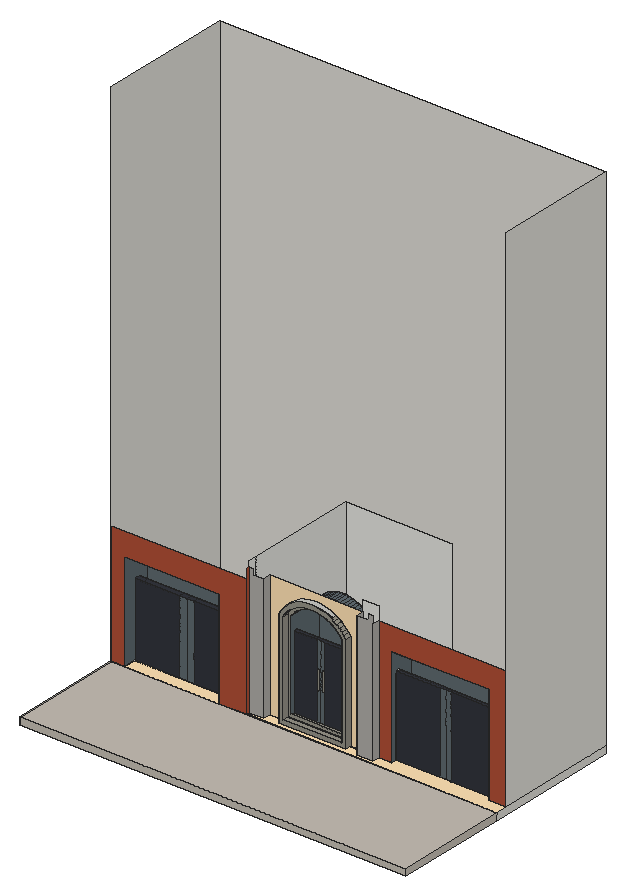
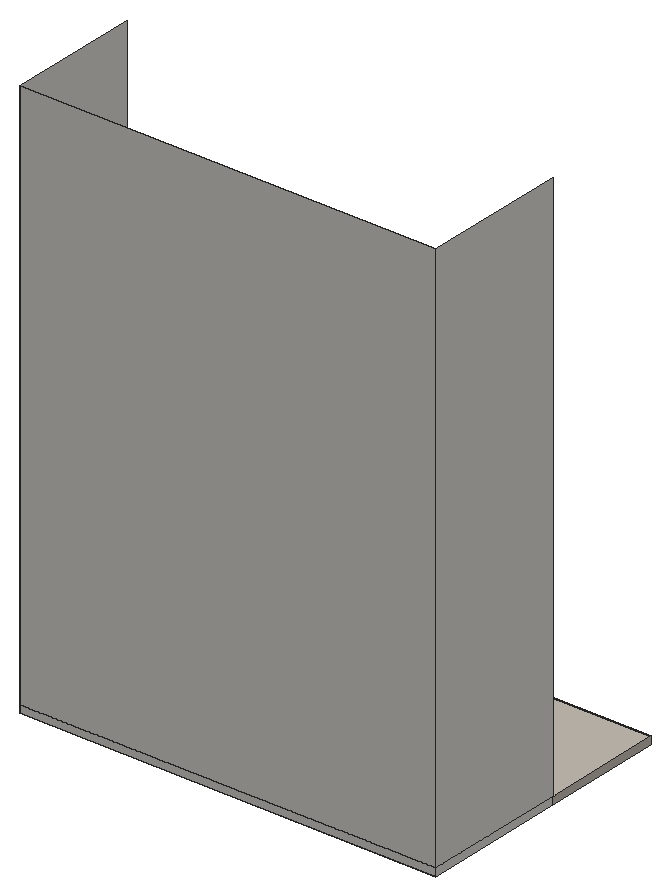
# SketchUp Ruby script. Lengths in inches.
U = 1.inch
M = Sketchup.active_model
def pt(a) = Geom::Point3d.new(a.map { |v| v * U })
def face(e, loops, mat)
  f = e.add_face(loops[0].map { |a| pt(a) })
  loops[1..].each { |l| e.add_face(l.map { |a| pt(a) }).erase! }
  f.material = f.back_material = mat if mat
  f
end
# faces: each face lists its corners as indices into pts; further lists are holes
def faces(e, pts, list, mat = nil) = list.each { |f| face(e, (f[0].is_a?(Array) ? f : [f]).map { |l| l.map { |i| pts[i] } }, mat) }
# xy, xz, yz: faces in a plane at the given z, y or x. An outline is a flat list of corners, or four numbers for a rectangle; further outlines are holes
def ring(l) = l.size == 4 ? [[l[0], l[1]], [l[2], l[1]], [l[2], l[3]], [l[0], l[3]]] : l.each_slice(2).to_a
def flat(e, list, mat, &to3) = list.each { |f| face(e, (f[0].is_a?(Array) ? f : [f]).map { |l| ring(l).map { |u, v| to3.(u, v) } }, mat) }
def xy(e, z, list, mat = nil) = flat(e, list, mat) { |x, y| [x, y, z] }
def xz(e, y, list, mat = nil) = flat(e, list, mat) { |x, z| [x, y, z] }
def yz(e, x, list, mat = nil) = flat(e, list, mat) { |y, z| [x, y, z] }
def lines(e, pts, list) = list.each { |a, b| e.add_line(pt(pts[a]), pt(pts[b])) }
# prism: a flat outline (further loops are holes) pulled along v
def prism(e, loops, v, mat = nil)
  f = face(e, loops, mat); d = Geom::Vector3d.new(v.map { |x| x * U })
  f.pushpull(f.normal.samedirection?(d) ? d.length : -d.length)
end
def box(e, o, s, mat = nil) = prism(e, [[o, [o[0] + s[0], o[1], o[2]], [o[0] + s[0], o[1] + s[1], o[2]], [o[0], o[1] + s[1], o[2]]]], [0, 0, s[2]], mat)
def at(x, y, z, deg = 0) = Geom::Transformation.translation(pt([x, y, z])) * Geom::Transformation.rotation(ORIGIN, Z_AXIS, deg.degrees)
def axes(o, x, y, z) = Geom::Transformation.new([*x, 0, *y, 0, *z, 0, *pt(o).to_a, 1])
def part(name) = M.definitions.add(name)
# library, detail: a bought-in or finely detailed component or shape, given as its bounding box
def library(name, o, s) = part(name).tap { |d| box(d.entities, o, s) }
def detail(e, o, s) = box(e.add_group.entities, o, s)
def put(e, d, t, mat = nil) = e.add_instance(d, t).tap { |i| i.material = mat if mat }
def group(e, t, mat = nil) = e.add_group.tap { |g| g.transformation = t; g.material = mat if mat }.entities
root = M.entities
M.materials.add("[Field Rectangle Tile]").color = [196, 189, 179]
M.materials.add("[Formica Beige]").color = [255, 225, 180]
M.materials.add("[Formica Graystone]").color = [149, 146, 135]
M.materials.add("[Formica Laminate Dark]").color = [50, 53, 60]
M.materials.add("[Formica Speckled Grey]").color = [94, 105, 111]
M.materials.add("[Rough Square Concrete Block]").color = [175, 79, 54]
M.materials.add("[Terrazzo Tile Light]").color = [173, 171, 166]
M.materials.add("[Terrazzo Tile Light]1").color = [219, 217, 210]
xy(root,0,[[10.25,0,499.12,144.04],[10.25,144.04,10.25,315.41,499.12,315.41,499.12,144.04,146.29,144.04,146.29,178.85,26.98,178.85,26.98,167.22,37.92,167.22,37.92,159.93,26.98,159.93,26.98,144.04],[26.98,144.04,146.29,159.93],[37.92,159.93,146.29,167.22],[26.98,167.22,146.29,178.85]])
xy(root,9,[[181.54,148.61,199.67,158.3],[317.75,148.61,338.35,158.3],[217.06,150.74,302.12,158.3],[181.54,158.3,181.54,301.14,315.73,301.14,338.35,158.3],[338.35,158.3,315.73,301.14,449.92,301.14,449.92,187.55,354.68,187.55,354.68,158.3],
  [354.68,164.83,476.62,168.86],[354.68,168.86,476.62,187.55]])
xy(root,9,[[10.25,0,499.12,144.04]],"[Field Rectangle Tile]")
xy(root,9,[[26.98,144.04,146.29,159.93],[181.54,144.04,499.12,144.04,499.12,158.3,476.62,158.3,476.62,164.83,354.68,164.83,354.68,158.3,338.35,158.3,338.35,148.61,317.75,148.61,317.75,158.3,302.12,158.3,302.12,150.74,217.06,150.74,217.06,158.3,199.67,158.3,199.67,148.61,181.54,148.61]],"[Formica Beige]")
xy(root,14.32,[[222.38,150.74,296.8,158.3]],"[Formica Graystone]")
xy(root,18.89,[[226.95,162.48,292.23,167.24],[226.95,167.24,292.23,201.93]])
xy(root,18.89,[[226.95,158.3,292.23,162.48]],"[Formica Graystone]")
xy(root,102.4375,[[26.98,159.93,37.92,167.22],[37.92,159.93,84.13,167.22],[84.13,159.93,93.02,167.22],[93.02,159.93,101.91,167.22],[101.91,159.93,146.29,167.22]],"[Formica Laminate Dark]")
xy(root,110.3125,[[354.68,164.83,410.3,168.86],[410.3,164.83,417.3,168.86],[417.3,164.83,424.29,168.86],[424.29,164.83,476.62,168.86]],"[Formica Laminate Dark]")
xy(root,112.08,[[226.95,162.48,292.23,167.24]],"[Formica Laminate Dark]")
xy(root,133.125,[[26.98,144.04,146.29,178.85]],"[Formica Speckled Grey]")
xy(root,134.875,[[354.68,158.3,476.62,187.55]],"[Formica Speckled Grey]")
xz(root,0,[[10.25,0,499.12,9]],"[Field Rectangle Tile]")
xz(root,144.04,[[10.25,0,26.98,9],[26.98,0,146.29,9],[146.29,0,181.54,9],[181.54,0,499.12,9]])
xz(root,144.04,[[10.25,9,26.98,9,26.98,133.125,146.29,133.125,146.29,9,181.54,9,181.54,162.44,10.25,162.44]],"[Rough Square Concrete Block]")
xz(root,148.61,[[181.54,9,199.67,9,199.67,167.08,186.17,167.08,186.17,174.01,181.54,174.01],[317.75,9,338.35,9,338.35,174.01,332.68,174.01,332.68,167.08,317.75,167.08]],"[Terrazzo Tile Light]")
xz(root,150.74,[[[217.06,9,302.12,9,302.12,132.93,299.7,136.43,297,139.71,294.05,142.77,290.86,145.58,287.46,148.125,283.86,150.39,280.1,152.36,276.18,154.02,272.15,155.36,268.02,156.37,263.83,157.04,259.59,157.38,255.28,157.35,250.99,156.91,246.77,156.08,242.64,154.85,238.64,153.25,234.81,151.28,231.17,148.96,227.77,146.3125,224.64,143.36,221.79,140.125,219.26,136.64,217.06,132.93],[222.38,14.32,222.38,131.48,223.7,133.71,225.95,136.8,228.46,139.66,231.24,142.27,234.25,144.61,237.46,146.66,240.85,148.41,244.39,149.82,248.04,150.91,251.78,151.64,255.57,152.03,259.4,152.06,263.19,151.76,266.97,151.15,270.68,150.24,274.3,149.04,277.82,147.54,281.21,145.77,284.45,143.74,287.51,141.45,290.37,138.92,293.03,136.17,295.45,133.22,296.8,131.27,296.8,14.32]]],"[Formica Graystone]")
xz(root,158.3,[[[217.06,9,217.06,132.93,219.26,136.64,221.79,140.125,224.64,143.36,227.77,146.3125,231.17,148.96,234.81,151.28,238.64,153.25,242.64,154.85,246.77,156.08,250.99,156.91,255.28,157.35,259.59,157.38,263.83,157.04,268.02,156.37,272.15,155.36,276.18,154.02,280.1,152.36,283.86,150.39,287.46,148.125,290.86,145.58,294.05,142.77,297,139.71,299.7,136.43,302.12,132.93,302.12,9],[222.38,14.32,296.8,14.32,296.8,131.27,295.45,133.22,293.03,136.17,290.37,138.92,287.51,141.45,284.45,143.74,281.21,145.77,277.82,147.54,274.3,149.04,270.68,150.24,266.97,151.15,263.19,151.76,259.4,152.06,255.57,152.03,251.78,151.64,248.04,150.91,244.39,149.82,240.85,148.41,237.46,146.66,234.25,144.61,231.24,142.27,228.46,139.66,225.95,136.8,223.7,133.71,222.38,131.48]],[317.75,9,338.35,180.875]])
xz(root,158.3,[[199.67,9,217.06,9,217.06,132.93,219.26,136.64,221.79,140.125,224.64,143.36,227.77,146.3125,231.17,148.96,234.81,151.28,238.64,153.25,242.64,154.85,246.77,156.08,250.99,156.91,255.28,157.35,259.59,157.38,263.83,157.04,268.02,156.37,272.15,155.36,276.18,154.02,280.1,152.36,283.86,150.39,287.46,148.125,290.86,145.58,294.05,142.77,297,139.71,299.7,136.43,302.12,132.93,302.12,9,317.75,9,317.75,167.08,199.67,167.08]],"[Formica Beige]")
xz(root,158.3,[[[222.38,14.32,296.8,14.32,296.8,131.27,295.45,133.22,293.03,136.17,290.37,138.92,287.51,141.45,284.45,143.74,281.21,145.77,277.82,147.54,274.3,149.04,270.68,150.24,266.97,151.15,263.19,151.76,259.4,152.06,255.57,152.03,251.78,151.64,248.04,150.91,244.39,149.82,240.85,148.41,237.46,146.66,234.25,144.61,231.24,142.27,228.46,139.66,225.95,136.8,223.7,133.71,222.38,131.48],[226.95,18.89,226.95,130.22,227.53,131.2,229.52,133.93,231.76,136.47,234.22,138.79,236.89,140.87,239.74,142.69,242.75,144.24,245.89,145.5,249.13,146.46,252.45,147.12,255.82,147.46,259.24,147.48,262.65,147.21,266.06,146.66,269.41,145.84,272.6875,144.75,275.87,143.41,278.93,141.81,281.85,139.97,284.62,137.9,287.21,135.61,289.61,133.13,291.8,130.46,292.23,129.84,292.23,18.89]]],"[Formica Graystone]")
xz(root,158.3,[[338.35,9,354.68,9,354.68,134.875,476.62,134.875,476.62,9,499.12,9,499.12,164.1875,338.35,164.1875]],"[Rough Square Concrete Block]")
xz(root,159.93,[[26.98,0,37.92,9],[37.92,0,84.13,9],[84.13,0,93.02,9],[93.02,0,101.91,9],[101.91,0,146.29,9]])
xz(root,159.93,[[26.98,9,84.13,102.4375],[101.91,9,146.29,102.4375]],"[Formica Laminate Dark]")
xz(root,159.93,[[84.13,9,93.02,102.4375],[93.02,9,101.91,102.4375]],"[Formica Speckled Grey]")
xz(root,162.48,[[256.66,54.69,258.98,78.94],[263.04,54.69,265.35,78.94]],"[Formica Graystone]")
xz(root,162.48,[[226.95,18.89,255.7,112.08],[266.32,18.89,292.23,112.08]],"[Formica Laminate Dark]")
xz(root,162.48,[[[255.7,18.89,261.3,112.08],[256.66,54.69,258.98,78.94]],[[261.3,18.89,266.32,112.08],[263.04,54.69,265.35,78.94]]],"[Formica Speckled Grey]")
xz(root,164.83,[[354.68,9,410.3,110.3125],[424.29,9,476.62,110.3125]],"[Formica Laminate Dark]")
xz(root,164.83,[[410.3,9,417.3,110.3125],[417.3,9,424.29,110.3125]],"[Formica Speckled Grey]")
xz(root,167.22,[[26.98,0,37.92,102.4375]])
xz(root,167.22,[[37.92,0,146.29,102.4375]],"[Formica Laminate Dark]")
xz(root,167.24,[[226.95,18.89,292.23,112.08]],"[Formica Laminate Dark]")
xz(root,168.86,[[354.68,9,476.62,110.3125]],"[Formica Laminate Dark]")
xz(root,178.85,[[26.98,0,146.29,133.125]],"[Formica Speckled Grey]")
xz(root,187.55,[[354.68,9,476.62,134.875]],"[Formica Speckled Grey]")
xz(root,201.93,[[226.95,18.89,292.23,18.89,292.23,129.84,291.8,130.46,289.61,133.13,287.21,135.61,284.62,137.9,281.85,139.97,278.93,141.81,275.87,143.41,272.6875,144.75,269.41,145.84,266.06,146.66,262.65,147.21,259.24,147.48,255.82,147.46,252.45,147.12,249.13,146.46,245.89,145.5,242.75,144.24,239.74,142.69,236.89,140.87,234.22,138.79,231.76,136.47,229.52,133.93,227.53,131.2,226.95,130.22]],"[Formica Speckled Grey]")
xz(root,301.14,[[181.54,9,315.73,180.875]])
xz(root,315.41,[[10.25,0,499.12,9],[10.25,9,499.12,660.875]],"[Terrazzo Tile Light]1")
yz(root,10.25,[[0,0,144.04,9]],"[Field Rectangle Tile]")
yz(root,10.25,[[144.04,0,315.41,9],[144.04,9,315.41,660.875]],"[Terrazzo Tile Light]1")
yz(root,26.98,[[144.04,0,159.93,9]])
yz(root,26.98,[[167.22,0,178.85,0,178.85,133.125,144.04,133.125,144.04,9,159.93,9,159.93,102.4375,167.22,102.4375]],"[Formica Speckled Grey]")
yz(root,146.29,[[144.04,0,159.93,9],[159.93,0,167.22,102.4375]])
yz(root,146.29,[[167.22,0,167.22,102.4375,159.93,102.4375,159.93,9,144.04,9,144.04,133.125,178.85,133.125,178.85,0]],"[Formica Speckled Grey]")
yz(root,181.54,[[148.61,9,158.3,180.875],[158.3,9,301.14,180.875]])
yz(root,181.54,[[144.04,9,148.61,174.01]],"[Rough Square Concrete Block]")
yz(root,199.67,[[148.61,9,158.3,167.08]],"[Terrazzo Tile Light]")
yz(root,217.06,[[150.74,9,158.3,132.93]],"[Formica Graystone]")
yz(root,222.38,[[150.74,14.32,158.3,131.48]],"[Formica Graystone]")
yz(root,226.95,[[162.48,18.89,167.24,112.08]])
yz(root,226.95,[[158.3,18.89,162.48,18.89,162.48,112.08,167.24,112.08,167.24,18.89,201.93,18.89,201.93,130.22,158.3,130.22]],"[Formica Speckled Grey]")
yz(root,292.23,[[162.48,18.89,167.24,112.08]])
yz(root,292.23,[[158.3,18.89,158.3,129.84,201.93,129.84,201.93,18.89,167.24,18.89,167.24,112.08,162.48,112.08,162.48,18.89]],"[Formica Speckled Grey]")
yz(root,296.8,[[150.74,14.32,158.3,131.27]],"[Formica Graystone]")
yz(root,302.12,[[150.74,9,158.3,132.93]],"[Formica Graystone]")
yz(root,317.75,[[148.61,9,158.3,167.08]],"[Terrazzo Tile Light]")
yz(root,338.35,[[148.61,9,158.3,164.1875]],"[Terrazzo Tile Light]")
yz(root,354.68,[[164.83,9,168.86,110.3125]])
yz(root,354.68,[[158.3,9,164.83,9,164.83,110.3125,168.86,110.3125,168.86,9,187.55,9,187.55,134.875,158.3,134.875]],"[Formica Speckled Grey]")
yz(root,476.62,[[164.83,9,168.86,110.3125]])
yz(root,476.62,[[158.3,9,158.3,134.875,187.55,134.875,187.55,9,168.86,9,168.86,110.3125,164.83,110.3125,164.83,9]],"[Formica Speckled Grey]")
yz(root,499.12,[[0,0,144.04,9]],"[Field Rectangle Tile]")
yz(root,499.12,[[144.04,0,315.41,9],[158.3,9,315.41,660.875]],"[Terrazzo Tile Light]1")
p = [[292.23,158.3,129.84],[291.8,158.3,130.46],[291.8,201.93,130.46],[292.23,201.93,129.84],[227.53,158.3,131.2],[226.95,158.3,130.22],
  [226.95,201.93,130.22],[227.53,201.93,131.2],[289.61,158.3,133.13],[289.61,201.93,133.13],[229.52,158.3,133.93],[229.52,201.93,133.93],
  [295.45,158.3,133.22],[296.8,158.3,131.27],[296.8,150.74,131.27],[295.45,150.74,133.22],[222.38,158.3,131.48],[223.7,158.3,133.71],
  [223.7,150.74,133.71],[222.38,150.74,131.48],[219.26,158.3,136.64],[217.06,158.3,132.93],[217.06,150.74,132.93],[219.26,150.74,136.64],
  [302.12,158.3,132.93],[299.7,158.3,136.43],[299.7,150.74,136.43],[302.12,150.74,132.93],[287.21,158.3,135.61],[287.21,201.93,135.61],
  [293.03,158.3,136.17],[293.03,150.74,136.17],[225.95,158.3,136.8],[225.95,150.74,136.8],[231.76,158.3,136.47],[231.76,201.93,136.47],
  [284.62,158.3,137.9],[284.62,201.93,137.9],[290.37,158.3,138.92],[290.37,150.74,138.92],[297,158.3,139.71],[297,150.74,139.71],
  [234.22,158.3,138.79],[234.22,201.93,138.79],[221.79,158.3,140.125],[221.79,150.74,140.125],[228.46,158.3,139.66],[228.46,150.74,139.66],
  [281.85,158.3,139.97],[281.85,201.93,139.97],[236.89,158.3,140.87],[236.89,201.93,140.87],[287.51,158.3,141.45],[287.51,150.74,141.45],
  [231.24,158.3,142.27],[231.24,150.74,142.27],[294.05,158.3,142.77],[294.05,150.74,142.77],[278.93,158.3,141.81],[278.93,201.93,141.81],
  [224.64,158.3,143.36],[224.64,150.74,143.36],[239.74,158.3,142.69],[239.74,201.93,142.69],[284.45,158.3,143.74],[284.45,150.74,143.74],
  [275.87,158.3,143.41],[275.87,201.93,143.41],[234.25,158.3,144.61],[234.25,150.74,144.61],[242.75,158.3,144.24],[242.75,201.93,144.24],
  [290.86,158.3,145.58],[290.86,150.74,145.58],[227.77,158.3,146.3125],[227.77,150.74,146.3125],[272.6875,158.3,144.75],[272.6875,201.93,144.75],
  [281.21,158.3,145.77],[281.21,150.74,145.77],[245.89,158.3,145.5],[245.89,201.93,145.5],[237.46,158.3,146.66],[237.46,150.74,146.66],
  [269.41,158.3,145.84],[269.41,201.93,145.84],[249.13,158.3,146.46],[249.13,201.93,146.46],[287.46,158.3,148.125],[287.46,150.74,148.125],
  [277.82,158.3,147.54],[277.82,150.74,147.54],[266.06,158.3,146.66],[266.06,201.93,146.66],[231.17,158.3,148.96],[231.17,150.74,148.96],
  [252.45,158.3,147.12],[252.45,201.93,147.12],[240.85,158.3,148.41],[240.85,150.74,148.41],[262.65,158.3,147.21],[262.65,201.93,147.21],
  [255.82,158.3,147.46],[255.82,201.93,147.46],[259.24,158.3,147.48],[259.24,201.93,147.48],[274.3,158.3,149.04],[274.3,150.74,149.04],
  [283.86,158.3,150.39],[283.86,150.74,150.39],[244.39,158.3,149.82],[244.39,150.74,149.82],[24.51,301.14,9],[24.51,144.04,9],
  [181.54,301.14,9],[24.51,301.14,180.875]]
faces(root,p,[[0,1,2,3],[4,5,6,7],[1,8,9,2],[10,4,7,11],[8,28,29,9],[34,10,11,35],[28,36,37,29],[42,34,35,43],
  [36,48,49,37],[50,42,43,51],[48,58,59,49],[62,50,51,63],[58,66,67,59],[70,62,63,71],[66,76,77,67],[80,70,71,81],
  [76,84,85,77],[86,80,81,87],[84,92,93,85],[96,86,87,97],[92,100,101,93],[102,96,97,103],[100,104,105,101],[104,102,103,105]],"[Formica Speckled Grey]")
faces(root,p,[[12,13,14,15],[16,17,18,19],[20,21,22,23],[24,25,26,27],[30,12,15,31],[17,32,33,18],[38,30,31,39],[25,40,41,26],
  [44,20,23,45],[32,46,47,33],[52,38,39,53],[46,54,55,47],[40,56,57,41],[60,44,45,61],[64,52,53,65],[54,68,69,55],
  [56,72,73,57],[74,60,61,75],[78,64,65,79],[68,82,83,69],[72,88,89,73],[90,78,79,91],[94,74,75,95],[82,98,99,83],
  [106,90,91,107],[88,108,109,89],[98,110,111,99]],"[Formica Graystone]")
lines(root,p,[[112,113],[114,112],[112,115]])
